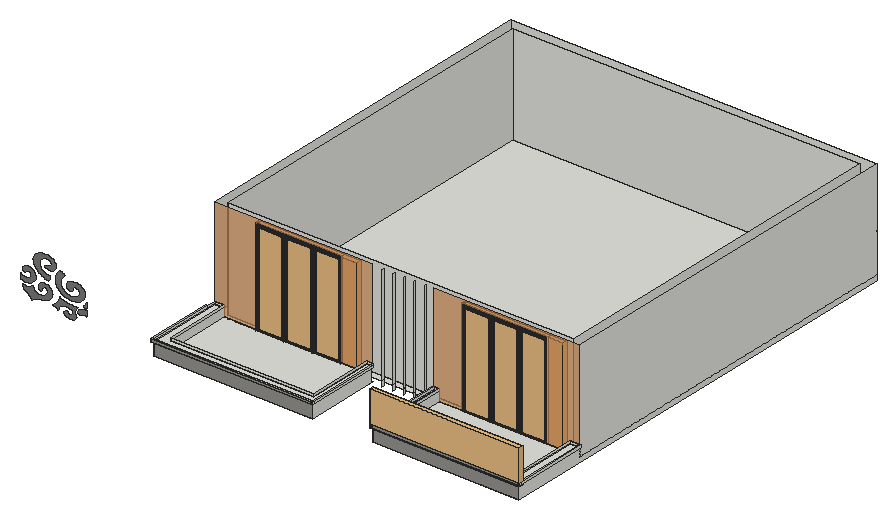
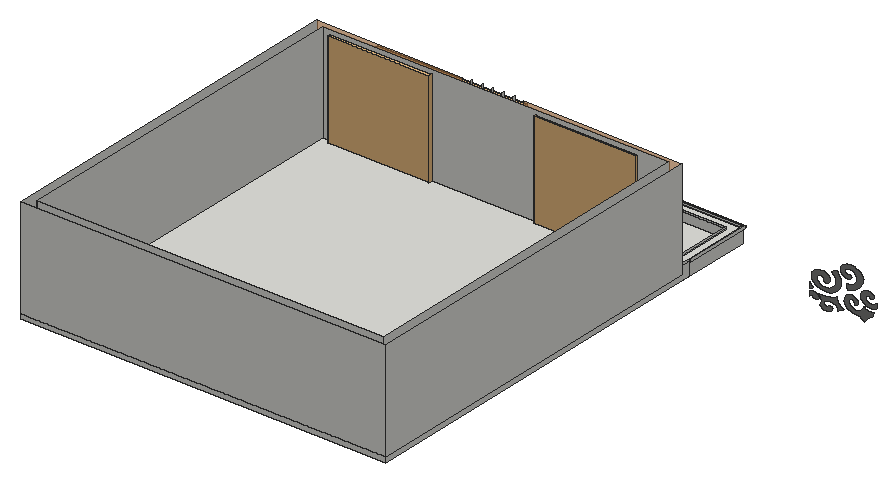
# SketchUp Ruby script. Lengths in inches.
U = 1.inch
M = Sketchup.active_model
def pt(a) = Geom::Point3d.new(a.map { |v| v * U })
def face(e, loops, mat)
  f = e.add_face(loops[0].map { |a| pt(a) })
  loops[1..].each { |l| e.add_face(l.map { |a| pt(a) }).erase! }
  f.material = f.back_material = mat if mat
  f
end
# faces: each face lists its corners as indices into pts; further lists are holes
def faces(e, pts, list, mat = nil) = list.each { |f| face(e, (f[0].is_a?(Array) ? f : [f]).map { |l| l.map { |i| pts[i] } }, mat) }
# xy, xz, yz: faces in a plane at the given z, y or x. An outline is a flat list of corners, or four numbers for a rectangle; further outlines are holes
def ring(l) = l.size == 4 ? [[l[0], l[1]], [l[2], l[1]], [l[2], l[3]], [l[0], l[3]]] : l.each_slice(2).to_a
def flat(e, list, mat, &to3) = list.each { |f| face(e, (f[0].is_a?(Array) ? f : [f]).map { |l| ring(l).map { |u, v| to3.(u, v) } }, mat) }
def xy(e, z, list, mat = nil) = flat(e, list, mat) { |x, y| [x, y, z] }
def xz(e, y, list, mat = nil) = flat(e, list, mat) { |x, z| [x, y, z] }
def yz(e, x, list, mat = nil) = flat(e, list, mat) { |y, z| [x, y, z] }
def lines(e, pts, list) = list.each { |a, b| e.add_line(pt(pts[a]), pt(pts[b])) }
# prism: a flat outline (further loops are holes) pulled along v
def prism(e, loops, v, mat = nil)
  f = face(e, loops, mat); d = Geom::Vector3d.new(v.map { |x| x * U })
  f.pushpull(f.normal.samedirection?(d) ? d.length : -d.length)
end
def box(e, o, s, mat = nil) = prism(e, [[o, [o[0] + s[0], o[1], o[2]], [o[0] + s[0], o[1] + s[1], o[2]], [o[0], o[1] + s[1], o[2]]]], [0, 0, s[2]], mat)
def at(x, y, z, deg = 0) = Geom::Transformation.translation(pt([x, y, z])) * Geom::Transformation.rotation(ORIGIN, Z_AXIS, deg.degrees)
def axes(o, x, y, z) = Geom::Transformation.new([*x, 0, *y, 0, *z, 0, *pt(o).to_a, 1])
def part(name) = M.definitions.add(name)
# library, detail: a bought-in or finely detailed component or shape, given as its bounding box
def library(name, o, s) = part(name).tap { |d| box(d.entities, o, s) }
def detail(e, o, s) = box(e.add_group.entities, o, s)
def put(e, d, t, mat = nil) = e.add_instance(d, t).tap { |i| i.material = mat if mat }
def group(e, t, mat = nil) = e.add_group.tap { |g| g.transformation = t; g.material = mat if mat }.entities
root = M.entities
M.materials.add("Wine2").color = [0, 0, 0]
M.materials["Wine2"].alpha = 0
M.materials.add("[0043_SaddleBrown]4").color = [124, 123, 122]
M.materials.add("[0130_Gainsboro]").color = [39, 45, 50]
M.materials.add("[Granite Light Gray]").color = [149, 148, 144]
M.materials.add("[Wood Floor Light]").color = [204, 176, 127]
M.materials.add("[Wood Floor]").color = [224, 152, 88]
M.materials["[Wood Floor]"].alpha = 0.68
c1 = part("Framed glazing panel")
xy(c1.entities,0,[[0,-0.98,43.07,0],[0,0,43.07,1.4]],"[0130_Gainsboro]")
xy(c1.entities,0.3,[[0.3,-1.43,42.77,-0.98]],"[0130_Gainsboro]")
xy(c1.entities,2.95,[[2.95,-1.43,40.12,-0.63],[2.95,-0.63,40.12,0],[2.95,0,40.12,0.64],[2.95,0.64,40.12,1.4]],"[0130_Gainsboro]")
xy(c1.entities,3.54,[[3.54,-0.63,39.53,0],[3.54,0,39.53,0.64]],"[0130_Gainsboro]")
xy(c1.entities,111.8125,[[3.54,-0.63,39.53,0],[3.54,0,39.53,0.64]],"[0130_Gainsboro]")
xy(c1.entities,112.4,[[2.95,-1.43,40.12,-0.63],[2.95,-0.63,40.12,0],[2.95,0,40.12,0.64],[2.95,0.64,40.12,1.4]],"[0130_Gainsboro]")
xy(c1.entities,115.05,[[0.3,-1.43,42.77,-0.98]],"[0130_Gainsboro]")
xy(c1.entities,115.35,[[0,-0.98,43.07,0],[0,0,43.07,1.4]],"[0130_Gainsboro]")
xz(c1.entities,-1.43,[[[0.3,0.3,42.77,115.05],[2.95,2.95,40.12,112.4]]],"[0130_Gainsboro]")
xz(c1.entities,-0.98,[[[0,0,43.07,115.35],[0.3,0.3,42.77,115.05]]],"[0130_Gainsboro]")
xz(c1.entities,-0.63,[[[2.95,2.95,40.12,112.4],[3.54,3.54,39.53,111.8125]]],"[0130_Gainsboro]")
xz(c1.entities,0,[[3.54,3.54,39.53,111.8125]],"Wine2")
xz(c1.entities,0,[[[0,0,43.07,115.35],[2.95,2.95,40.12,112.4]],[[2.95,2.95,40.12,112.4],[3.54,3.54,39.53,111.8125]]],"[0130_Gainsboro]")
xz(c1.entities,0.64,[[[2.95,2.95,40.12,112.4],[3.54,3.54,39.53,111.8125]]],"[0130_Gainsboro]")
xz(c1.entities,1.4,[[[0,0,43.07,115.35],[2.95,2.95,40.12,112.4]]],"[0130_Gainsboro]")
yz(c1.entities,0,[[-0.98,0,0,115.35],[0,0,1.4,115.35]],"[0130_Gainsboro]")
yz(c1.entities,0.3,[[-1.43,0.3,-0.98,115.05]],"[0130_Gainsboro]")
yz(c1.entities,2.95,[[-1.43,2.95,-0.63,112.4],[-0.63,2.95,0,112.4],[0,2.95,0.64,112.4],[0.64,2.95,1.4,112.4]],"[0130_Gainsboro]")
yz(c1.entities,3.54,[[-0.63,3.54,0,111.8125],[0,3.54,0.64,111.8125]],"[0130_Gainsboro]")
yz(c1.entities,39.53,[[-0.63,3.54,0,111.8125],[0,3.54,0.64,111.8125]],"[0130_Gainsboro]")
yz(c1.entities,40.12,[[-1.43,2.95,-0.63,112.4],[-0.63,2.95,0,112.4],[0,2.95,0.64,112.4],[0.64,2.95,1.4,112.4]],"[0130_Gainsboro]")
yz(c1.entities,42.77,[[-1.43,0.3,-0.98,115.05]],"[0130_Gainsboro]")
yz(c1.entities,43.07,[[-0.98,0,0,115.35],[0,0,1.4,115.35]],"[0130_Gainsboro]")
c2 = part("Glazing assembly")
put(c2.entities,c1,axes([90.57,1.43,0],[1.05148,0,0],[0,1,0],[0,0,1]))
put(c2.entities,c1,axes([0,1.43,0],[1.05148,0,0],[0,1,0],[0,0,1]))
put(c2.entities,c1,axes([45.29,1.43,0],[1.05148,0,0],[0,1,0],[0,0,1]))
c3 = library("Curtains",[0,0,0],[121.73,8.19,117.22])
c4 = library("Glass Railing",[0,0,0],[139.5,4.76,42])
xy(root,388.875,[[4353.89,651.03,4455.14,657.03],[4601.63,651.03,4702.88,657.03]])
xy(root,394.4375,[[4303.63,559.875,4494.32,570.83],[4566.77,559.875,4742.06,570.83],[4314.96,657.03,4730.74,1085.17]])
xy(root,394.4375,[[4303.63,570.83,4314.96,651.03],[4314.96,570.83,4494.32,651.03],[4566.77,570.83,4730.74,651.03],[4730.74,570.83,4742.06,651.03]],"[Wood Floor Light]")
xy(root,400.4375,[[4314.96,570.83,4486.46,570.83,4486.46,651.03,4455.14,651.03,4455.14,657.03,4353.89,657.03,4353.89,651.03,4314.96,651.03],[4572.84,570.83,4730.74,570.83,4730.74,651.03,4702.88,651.03,4702.88,657.03,4601.63,657.03,4601.63,651.03,4572.84,651.03],[4303.63,651.03,4303.63,1096.5,4742.06,1096.5,4742.06,651.03,4702.88,651.03,4702.88,657.03,4730.74,657.03,4730.74,1085.17,4314.96,1085.17,4314.96,657.03,4353.89,657.03,4353.89,651.03],[4314.96,657.03,4730.74,1085.17]])
xy(root,410.625,[[4301.88,557.9375,4494.32,559.875],[4494.32,557.9375,4496.26,559.875],[4564.83,557.9375,4566.77,559.875],[4566.77,557.9375,4742.06,559.875],[4742.06,557.9375,4744,559.875],
  [4301.7,559.875,4303.63,640.11],[4303.63,559.875,4303.63,651.03,4314.96,651.03,4314.96,570.83,4486.46,570.83,4486.46,651.03,4494.32,651.03,4494.32,559.875],[4494.32,559.875,4496.26,647.91],[4564.83,559.875,4566.77,651.03],[4566.77,559.875,4566.77,651.03,4572.84,651.03,4572.84,570.83,4730.74,570.83,4730.74,651.03,4742.06,651.03,4742.06,559.875],
  [4742.06,559.875,4744,651.03]])
xz(root,557.9375,[[4742.06,410.625,4744,413.5]])
xz(root,557.9375,[[4301.88,410.625,4494.32,413.5],[4494.32,410.625,4496.26,413.5],[4564.83,410.625,4566.77,413.5],[4566.77,410.625,4742.06,413.5]],"[Granite Light Gray]")
xz(root,559.875,[[4301.7,410.625,4301.88,413.5],[4301.88,410.625,4303.63,413.5],[4303.63,410.625,4494.32,413.5],[4494.32,410.625,4496.26,413.5],[4564.83,410.625,4566.77,413.5],
  [4566.77,410.625,4742.06,413.5],[4742.06,410.625,4744,413.5]])
xz(root,559.875,[[4303.63,394.4375,4494.32,410.625],[4566.77,394.4375,4742.06,410.625]],"[Granite Light Gray]")
xz(root,570.83,[[4314.96,400.4375,4486.46,410.625],[4572.84,400.4375,4730.74,410.625],[4314.96,410.625,4486.46,413.5],[4572.84,410.625,4730.74,413.5]])
xz(root,589.17,[[4179.4,378.34,4181.0625,378.37,4182.68,378.64,4184.1875,379.15,4185.52,379.86,4186.62,380.76,4187.44,381.8,4186.875,382.74,4186.43,383.71,4186.11,384.71,4185.9,385.72,4185.83,386.75,4185.88,387.77,4186.06,388.79,4186.36,389.79,4186.78,390.76,4187.32,391.71,4187.97,392.62,4188.74,393.48,4186.86,393.37,4184.97,393.33,4183.09,393.38,4181.21,393.5,4179.35,393.71,4177.5,393.99,4175.68,394.35,4173.9,394.79,4172.15,395.3,4170.45,395.88,4168.8,396.54,4167.2,397.26,4167.08,396.19,4166.85,395.13,4166.51,394.09,4166.07,393.07,4165.51,392.07,4164.86,391.11,4164.11,390.1875,4163.27,389.31,4162.33,388.47,4161.3125,387.69,4160.22,386.97,4159.05,386.31,4159.67,386.1,4160.28,385.89,4160.89,385.67,4161.48,385.44,4162.08,385.2,4163.24,384.7,4163.81,384.44,4164.38,384.16,4164.9375,383.88,4165.48,383.59,4166.02,383.3,4166.13,384.7,4166.66,386.05,4167.58,387.29,4168.85,388.35,4170.41,389.19,4172.19,389.77,4174.1,390.05,4176.05,390.03,4177.94,389.7,4179.69,389.08,4181.21,388.2,4182.43,387.11,4182.47,386.77,4182.49,386.43,4182.5,386.09,4182.49,385.75,4182.47,385.41,4182.43,385.07,4182.38,384.73,4182.32,384.39,4182.24,384.06,4182.15,383.72,4182.04,383.39,4181.92,383.06,4181.33,382.875,4180.7,382.76,4180.05,382.72,4179.41,382.75,4178.77,382.85,4178.17,383.03,4177.62,383.27,4177.13,383.58,4176.71,383.93,4176.37,384.33,4176.13,384.76,4175.98,385.22,4175.58,385.09,4175.1875,384.95,4174.81,384.79,4174.44,384.61,4174.09,384.41,4173.76,384.2,4173.45,383.98,4173.16,383.74,4172.89,383.48,4172.64,383.22,4172.42,382.95,4172.22,382.66,4172.8,381.54,4173.69,380.53,4174.85,379.68,4176.23,379.01,4177.77,378.55],[4133.84,382.25,4134.45,383.03,4135.16,383.77,4135.98,384.44,4136.89,385.06,4137.875,385.6,4138.9375,386.07,4140.06,386.46,4141.23,386.77,4142.44,386.98,4143.67,387.11,4144.92,387.15,4146.16,387.09,4148.58,387.5,4150.86,388.2,4152.94,389.18,4154.75,390.4,4156.24,391.84,4157.35,393.4375,4158.07,395.15,4158.35,396.93,4158.21,398.71,4157.63,400.46,4156.64,402.1,4155.27,403.59,4154.15,404.41,4152.8,405.05,4151.31,405.47,4149.72,405.65,4148.11,405.59,4146.5625,405.29,4145.14,404.75,4143.89,404.02,4142.9,403.11,4142.18,402.07,4141.79,400.95,4141.73,399.79,4141.79,399.43,4141.9,399.08,4142.07,398.73,4142.28,398.4,4142.53,398.09,4142.83,397.8,4143.17,397.53,4143.55,397.29,4143.96,397.08,4144.39,396.9,4144.85,396.75,4145.33,396.64,4145.41,397.15,4145.54,397.65,4145.7,398.15,4145.9,398.64,4146.15,399.13,4146.43,399.6,4146.75,400.06,4147.1,400.5,4147.49,400.93,4147.92,401.34,4148.375,401.74,4148.86,402.11,4149.8,401.77,4150.65,401.34,4151.4,400.81,4152.02,400.2,4152.51,399.54,4152.86,398.83,4153.04,398.08,4153.07,397.33,4152.93,396.58,4152.64,395.86,4152.19,395.18,4151.6,394.55,4150.77,393.61,4149.7,392.8,4148.44,392.14,4147.04,391.66,4145.54,391.38,4143.99,391.3,4142.45,391.43,4140.97,391.76,4139.6,392.28,4138.38,392.98,4137.37,393.82,4136.58,394.79,4136.37,395.05,4136.17,395.3125,4135.97,395.58,4135.79,395.85,4135.47,396.41,4135.33,396.69,4135.09,397.27,4134.99,397.5625,4134.9,397.86,4134.83,398.15,4134.13,397.49,4133.33,396.89,4132.44,396.375,4131.46,395.94,4130.41,395.6,4129.3125,395.35,4128.18,395.2,4127.03,395.16,4125.88,395.22,4124.75,395.38,4123.66,395.64,4122.625,396,4122.84,395.6875,4123.03,395.37,4123.2,395.04,4123.34,394.71,4123.45,394.375,4123.54,394.03,4123.6,393.6875,4123.63,393.34,4123.63,392.99,4123.61,392.65,4123.56,392.3,4123.48,391.96,4124.62,391.33,4125.72,390.67,4126.77,389.96,4127.78,389.22,4128.73,388.45,4129.63,387.64,4130.48,386.81,4131.27,385.95,4132.01,385.06,4132.68,384.14,4133.29,383.2],[4191.94,386.82,4192.48,386.85,4192.95,386.92,4193.4,387.02,4193.84,387.15,4194.26,387.31,4194.66,387.49,4195.03,387.7,4195.38,387.93,4195.7,388.18,4195.99,388.45,4196.24,388.74,4196.45,389.05,4196.63,389.36,4196.98,389.23,4197.3125,389.09,4197.65,388.93,4197.97,388.77,4198.59,388.43,4198.89,388.24,4199.18,388.05,4199.46,387.85,4199.73,387.65,4199.99,387.4375,4200.24,387.22,4200.24,393,4199.27,393.38,4198.22,393.65,4197.13,393.8,4196.02,393.8125,4194.92,393.7,4193.86,393.47,4192.87,393.11,4191.96,392.65,4191.17,392.09,4190.51,391.45,4190.01,390.73,4189.66,389.97,4189.41,389.63,4189.25,389.25,4189.2,388.86,4189.25,388.47,4189.4,388.09,4189.65,387.74,4189.99,387.4375,4190.41,387.18,4190.88,386.99,4191.4,386.87],[4199.86,396.46,4200.24,396.47,4200.24,402.56,4199.96,402.125,4199.67,401.6875,4199.36,401.26,4199.05,400.83,4198.72,400.41,4198.38,399.99,4198.03,399.58,4197.66,399.18,4197.29,398.77,4196.9,398.38,4196.5,397.99,4196.1,397.61,4196.37,397.42,4196.67,397.24,4196.98,397.08,4197.3,396.9375,4197.64,396.8125,4197.99,396.71,4198.35,396.62,4198.72,396.55,4199.1,396.5,4199.48,396.47],[4181.74,398.78,4183.94,398.88,4186.1,399.21,4188.18,399.74,4190.14,400.47,4191.95,401.39,4193.56,402.47,4194.96,403.7,4196.11,405.0625,4196.99,406.52,4197.59,408.05,4197.89,409.625,4197.89,410.99,4197.61,412.35,4197.05,413.65,4196.24,414.89,4195.18,416.03,4193.91,417.04,4192.44,417.91,4190.82,418.61,4189.07,419.14,4187.23,419.47,4185.34,419.61,4183.45,419.54,4181.97,419.33,4180.57,418.9375,4179.27,418.39,4178.12,417.7,4177.14,416.875,4176.36,415.95,4175.79,414.95,4175.47,413.89,4175.39,412.81,4175.55,411.73,4175.96,410.68,4176.6,409.7,4177.12,409.31,4177.73,409,4178.42,408.79,4179.16,408.68,4179.91,408.6875,4180.65,408.8,4181.34,409.03,4181.94,409.35,4182.45,409.75,4182.82,410.22,4183.06,410.73,4182.95,411.09,4182.89,411.45,4182.88,411.81,4182.9375,412.17,4183.05,412.52,4183.21,412.87,4183.43,413.19,4183.69,413.5,4184,413.79,4184.36,414.04,4184.75,414.27,4185.17,414.46,4186.18,414.36,4187.16,414.15,4188.08,413.83,4188.92,413.41,4189.66,412.9,4190.29,412.32,4190.78,411.68,4191.13,410.98,4191.33,410.26,4191.375,409.53,4191.26,408.8,4190.99,408.08,4190.25,406.9,4189.24,405.82,4187.99,404.88,4186.54,404.1,4184.9375,403.5,4183.22,403.11,4181.43,402.93,4179.62,402.96,4177.85,403.22,4176.16,403.68,4174.6,404.34,4173.22,405.17,4171.77,406.36,4170.55,407.66,4169.57,409.08,4168.87,410.57,4168.4375,412.12,4168.29,413.7,4168.4375,415.27,4168.87,416.82,4169.57,418.3125,4170.55,419.73,4171.77,421.04,4173.22,422.22,4172.86,422.57,4172.47,422.9,4172.07,423.22,4171.64,423.53,4171.2,423.82,4170.74,424.1,4170.26,424.37,4169.76,424.61,4169.25,424.84,4168.73,425.06,4168.19,425.25,4167.64,425.43,4166.52,424.36,4165.51,423.23,4164.62,422.04,4163.85,420.8125,4163.22,419.55,4162.71,418.25,4162.35,416.93,4162.11,415.6,4162.02,414.25,4162.07,412.91,4162.25,411.57,4162.57,410.24,4163.1,408.8125,4163.83,407.43,4164.75,406.1,4165.86,404.85,4167.13,403.69,4168.57,402.63,4170.14,401.68,4171.84,400.85,4173.65,400.15,4175.55,399.58,4177.52,399.16,4179.54,398.88],
  [4126.85,399.74,4127.92,399.78,4128.99,399.9,4130.03,400.1,4131.04,400.36,4132.01,400.7,4133.71,401.49,4135.21,402.47,4136.47,403.61,4137.46,404.88,4138.15,406.25,4138.54,407.68,4138.6,409.14,4138.33,410.58,4137.75,411.98,4136.87,413.29,4135.71,414.48,4134.29,415.52,4133.3125,416.12,4132.2,416.58,4130.98,416.875,4129.7,417,4128.42,416.95,4127.17,416.72,4126.01,416.33,4124.97,415.79,4124.08,415.12,4123.39,414.34,4122.92,413.48,4122.68,412.57,4122.59,412.22,4122.59,411.86,4122.7,411.51,4122.89,411.18,4123.17,410.89,4123.52,410.63,4123.93,410.4375,4124.39,410.3,4124.88,410.24,4125.375,410.24,4125.86,410.31,4126.32,410.45,4126.59,410.7,4126.875,410.9375,4127.18,411.17,4127.51,411.38,4127.86,411.58,4128.22,411.76,4128.6,411.92,4128.99,412.07,4129.39,412.2,4129.81,412.31,4130.23,412.4,4130.66,412.47,4131.22,412.12,4131.72,411.73,4132.15,411.29,4132.5,410.82,4132.77,410.32,4132.95,409.8,4133.04,409.27,4133.05,408.74,4132.96,408.2,4132.78,407.69,4132.51,407.1875,4132.16,406.71,4131.4375,406,4130.55,405.39,4129.54,404.89,4128.42,404.53,4127.23,404.3,4126.01,404.23,4124.78,404.3,4123.6,404.53,4122.48,404.89,4121.46,405.39,4120.58,406,4119.85,406.71,4119.85,401.47,4120.73,401.01,4121.66,400.625,4122.64,400.3,4123.66,400.05,4124.7,399.875,4125.77,399.77],[4153.875,409.96,4154.29,410.4,4154.65,410.87,4154.96,411.35,4155.23,411.86,4155.4375,412.37,4155.59,412.89,4155.69,413.42,4155.74,413.96,4155.73,414.49,4155.66,415.03,4155.54,415.56,4155.37,416.08,4154.01,415.96,4152.65,415.98,4151.31,416.14,4150.01,416.43,4148.78,416.85,4147.63,417.38,4146.61,418.02,4145.71,418.76,4144.96,419.58,4144.38,420.47,4143.97,421.4,4143.75,422.37,4143.38,423.29,4143.15,424.22,4143.0625,425.17,4143.12,426.125,4143.31,427.06,4143.64,427.99,4144.11,428.875,4144.7,429.73,4145.42,430.52,4146.26,431.26,4147.19,431.93,4148.23,432.53,4149.18,432.92,4150.23,433.1875,4151.32,433.3,4152.43,433.26,4153.5,433.08,4154.51,432.75,4155.41,432.29,4156.18,431.71,4156.78,431.04,4157.19,430.3,4157.41,429.52,4157.41,428.72,4157.32,428.33,4157.16,427.95,4156.93,427.59,4156.63,427.25,4156.28,426.95,4155.86,426.6875,4155.41,426.46,4154.91,426.29,4154.39,426.16,4153.85,426.09,4153.29,426.07,4152.74,426.11,4152.17,426.125,4151.61,426.05,4151.08,425.88,4150.62,425.63,4150.25,425.3125,4150,424.94,4149.86,424.54,4149.86,424.13,4149.98,423.72,4150.23,423.35,4150.59,423.03,4151.04,422.77,4152.29,422.33,4153.63,422.0625,4155.01,421.97,4156.39,422.0625,4157.73,422.33,4158.98,422.77,4160.09,423.37,4161.04,424.1,4161.78,424.95,4162.31,425.875,4162.58,426.86,4162.61,427.86,4162.66,429.07,4162.49,430.28,4162.08,431.45,4161.46,432.58,4160.625,433.63,4159.6,434.59,4158.4,435.44,4157.05,436.17,4155.58,436.75,4154.01,437.18,4152.37,437.46,4150.69,437.5625,4148.36,437.47,4146.07,437.11,4143.89,436.49,4141.87,435.64,4140.0625,434.58,4138.5,433.32,4137.24,431.9,4136.29,430.36,4135.69,428.73,4135.45,427.05,4135.58,425.37,4136.07,423.72,4136.625,422.12,4137.38,420.56,4138.33,419.06,4139.47,417.63,4140.79,416.28,4142.27,415.02,4143.91,413.87,4145.69,412.83,4147.59,411.91,4149.6,411.12,4151.7,410.47]],"[0043_SaddleBrown]4")
xz(root,640.11,[[4301.7,410.625,4303.63,413.5]])
xz(root,647.91,[[4494.32,410.625,4496.26,413.5]])
xz(root,651.03,[[4303.63,400.4375,4314.96,410.625],[4730.74,400.4375,4742.06,410.625],[4303.63,410.625,4314.96,413.5],[4486.46,410.625,4494.32,413.5],[4564.83,410.625,4566.56,413.5],
  [4566.56,410.625,4566.77,413.5],[4566.77,410.625,4572.84,413.5],[4730.74,410.625,4742.06,413.5],[4742.06,410.625,4744,413.5]])
xz(root,651.03,[[4314.96,400.4375,4353.89,400.4375,4353.89,514.875,4455.14,514.875,4455.14,400.4375,4486.46,400.4375,4486.46,413.5,4494.32,413.5,4494.32,520.4375,4303.63,520.4375,4303.63,413.5,4314.96,413.5],[4572.84,400.4375,4601.63,400.4375,4601.63,514.875,4702.88,514.875,4702.88,400.4375,4730.74,400.4375,4730.74,413.5,4742.06,413.5,4742.06,520.4375,4566.77,520.4375,4566.77,413.5,4572.84,413.5]],"[Wood Floor]")
xz(root,657.03,[[4314.96,400.4375,4314.96,520.4375,4730.74,520.4375,4730.74,400.4375,4702.88,400.4375,4702.88,514.875,4601.63,514.875,4601.63,400.4375,4455.14,400.4375,4455.14,514.875,4353.89,514.875,4353.89,400.4375]])
xz(root,1085.17,[[4314.96,400.4375,4730.74,520.4375]])
xz(root,1096.5,[[4303.63,394.4375,4742.06,400.4375],[4303.63,400.4375,4742.06,520.4375]])
yz(root,4301.7,[[559.875,410.625,640.11,413.5]])
yz(root,4301.88,[[557.9375,410.625,559.875,413.5]])
yz(root,4303.63,[[559.875,394.4375,640.11,410.625],[640.11,394.4375,640.11,410.625,651.03,410.625,651.03,400.4375,1096.5,400.4375,1096.5,394.4375],[651.03,400.4375,1096.5,520.4375],[559.875,410.625,640.11,413.5],[640.11,410.625,651.03,413.5]])
yz(root,4314.96,[[570.83,400.4375,651.03,410.625],[657.03,400.4375,1085.17,520.4375],[570.83,410.625,651.03,413.5]])
yz(root,4353.89,[[651.03,400.4375,657.03,514.875]])
yz(root,4455.14,[[651.03,400.4375,657.03,514.875]])
yz(root,4486.46,[[570.83,400.4375,651.03,410.625],[570.83,410.625,651.03,413.5]])
yz(root,4494.32,[[559.875,394.4375,647.91,410.625],[557.9375,410.625,559.875,413.5],[559.875,410.625,647.91,413.5],[647.91,410.625,651.03,413.5]])
yz(root,4496.26,[[557.9375,410.625,559.875,413.5],[559.875,410.625,647.91,413.5]])
yz(root,4507.32,[[647.91,394.4375,651.03,400.4375],[647.91,400.4375,651.03,520.4375]])
yz(root,4520.07,[[648.85,394.4375,651.03,400.4375],[648.85,400.4375,651.03,520.4375]])
yz(root,4532.19,[[648.85,394.4375,651.03,400.4375],[648.85,400.4375,651.03,520.4375]])
yz(root,4544.57,[[648.85,394.4375,651.03,400.4375],[648.85,400.4375,651.03,520.4375]])
yz(root,4557.44,[[648.85,394.4375,651.03,400.4375],[648.85,400.4375,651.03,520.4375]])
yz(root,4564.83,[[557.9375,410.625,559.875,413.5],[559.875,410.625,651.03,413.5]])
yz(root,4566.77,[[559.875,394.4375,651.03,410.625],[557.9375,410.625,559.875,413.5],[559.875,410.625,651.03,413.5]])
yz(root,4572.84,[[570.83,400.4375,651.03,410.625],[570.83,410.625,651.03,413.5]])
yz(root,4601.63,[[651.03,400.4375,657.03,514.875]])
yz(root,4702.88,[[651.03,400.4375,657.03,514.875]])
yz(root,4730.74,[[570.83,400.4375,651.03,410.625],[657.03,400.4375,1085.17,520.4375],[570.83,410.625,651.03,413.5]])
yz(root,4742.06,[[559.875,394.4375,1096.5,394.4375,1096.5,400.4375,651.03,400.4375,651.03,410.625,559.875,410.625],[651.03,400.4375,1096.5,520.4375],[557.9375,410.625,559.875,413.5],[559.875,410.625,651.03,413.5]])
yz(root,4744,[[557.9375,410.625,559.875,413.5],[559.875,410.625,651.03,413.5]])
p = [[4183.14,589.17,411.27],[4183.06,589.17,410.73]]
lines(root,p,[[0,1]])
put(root,c2,axes([4353.48,650.7,397.79],[0.75,0,0],[0,0.75,0],[0,0,1.01765]))
put(root,c3,at(4352.7,651.68,397.95))
put(root,c2,axes([4600.98,651.03,397.48],[0.75,0,0],[0,0.75,0],[0,0,1.01765]))
put(root,c4,axes([4564.83,558.12,409.93],[1.28434,0,0],[0,1,0],[0,0,1]),"[Granite Light Gray]")
put(root,c3,at(4599.74,652.22,397.95))
